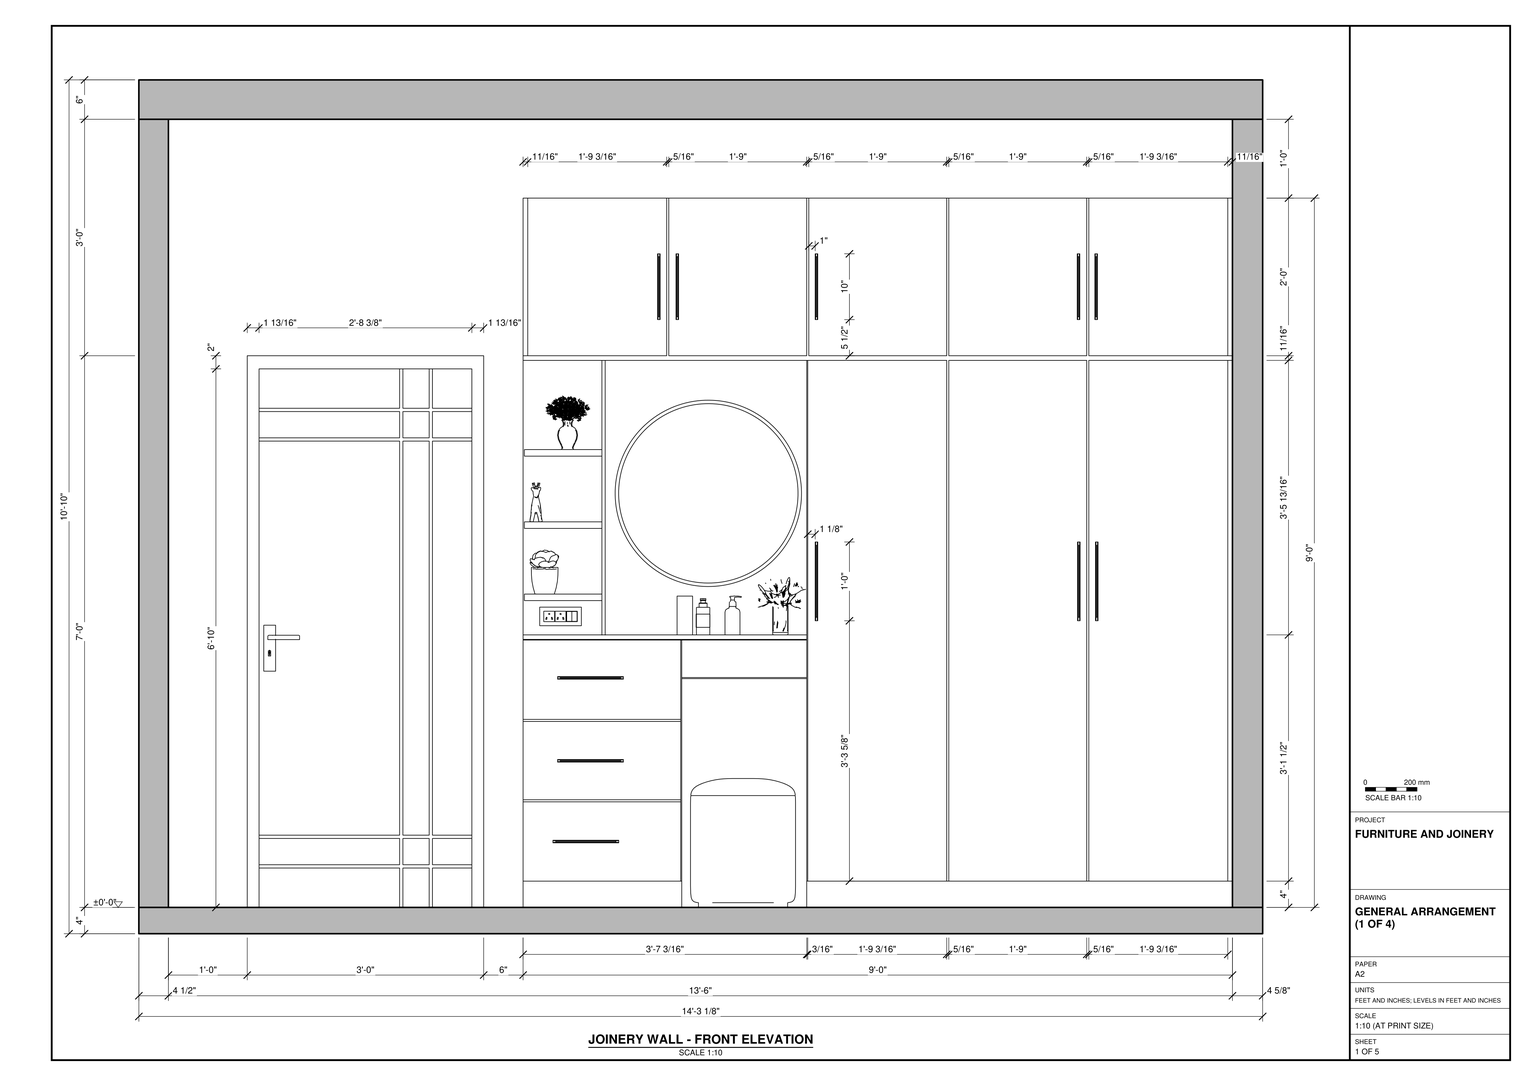
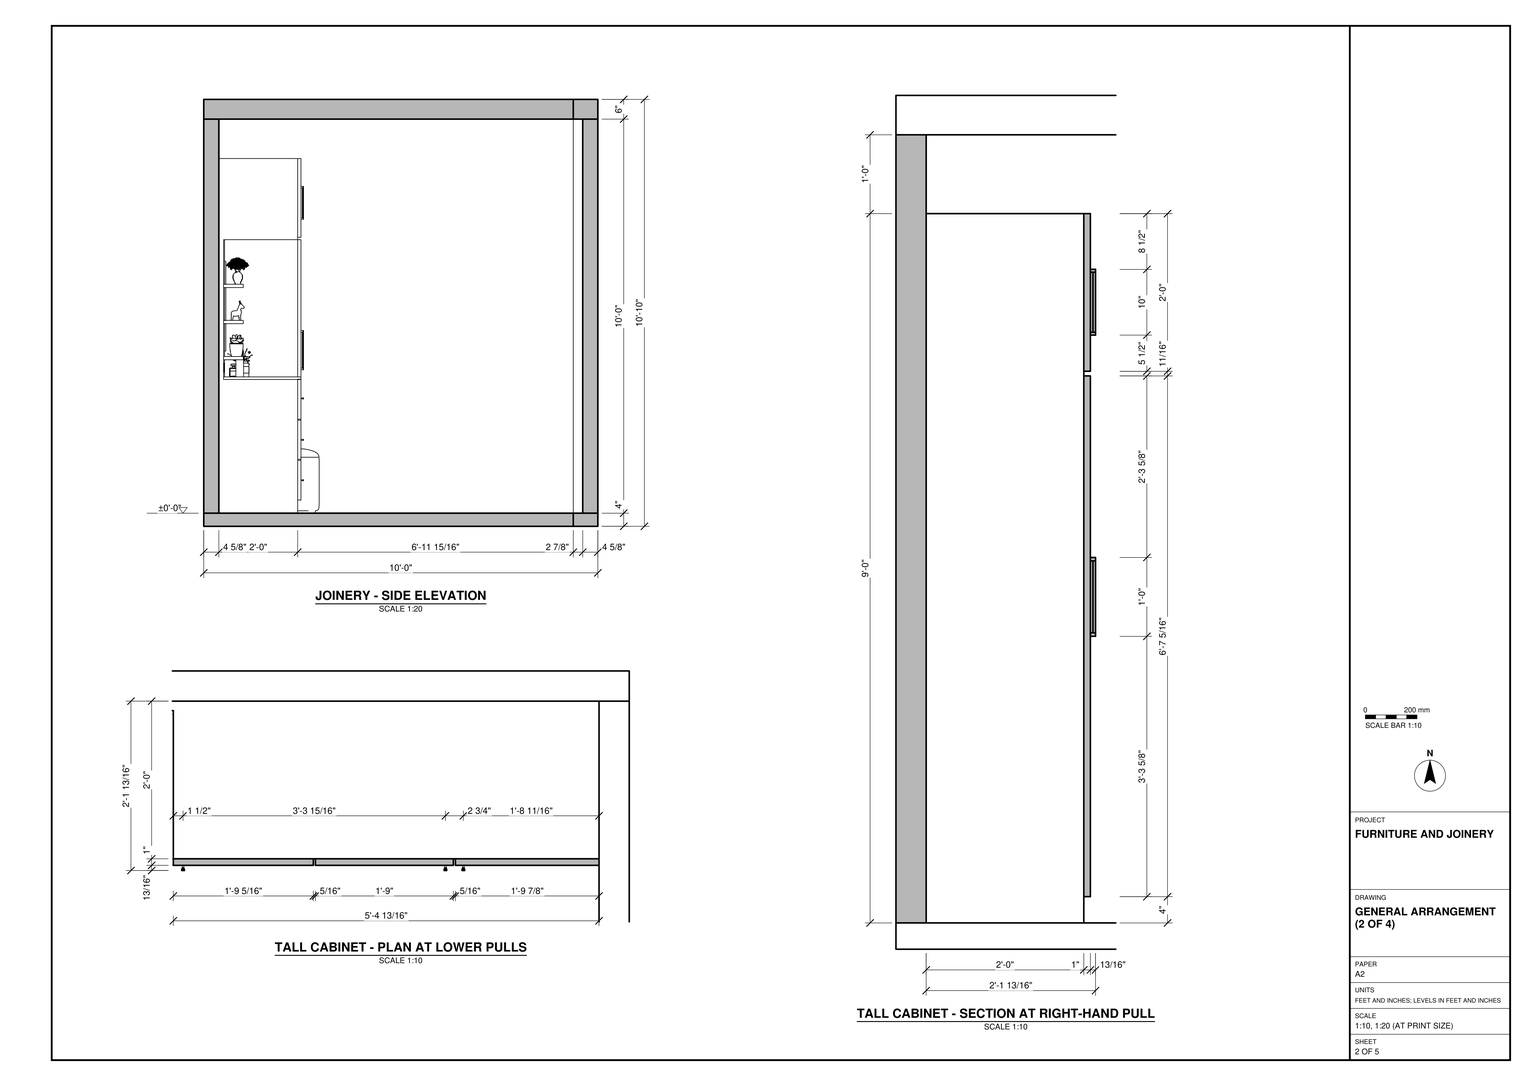
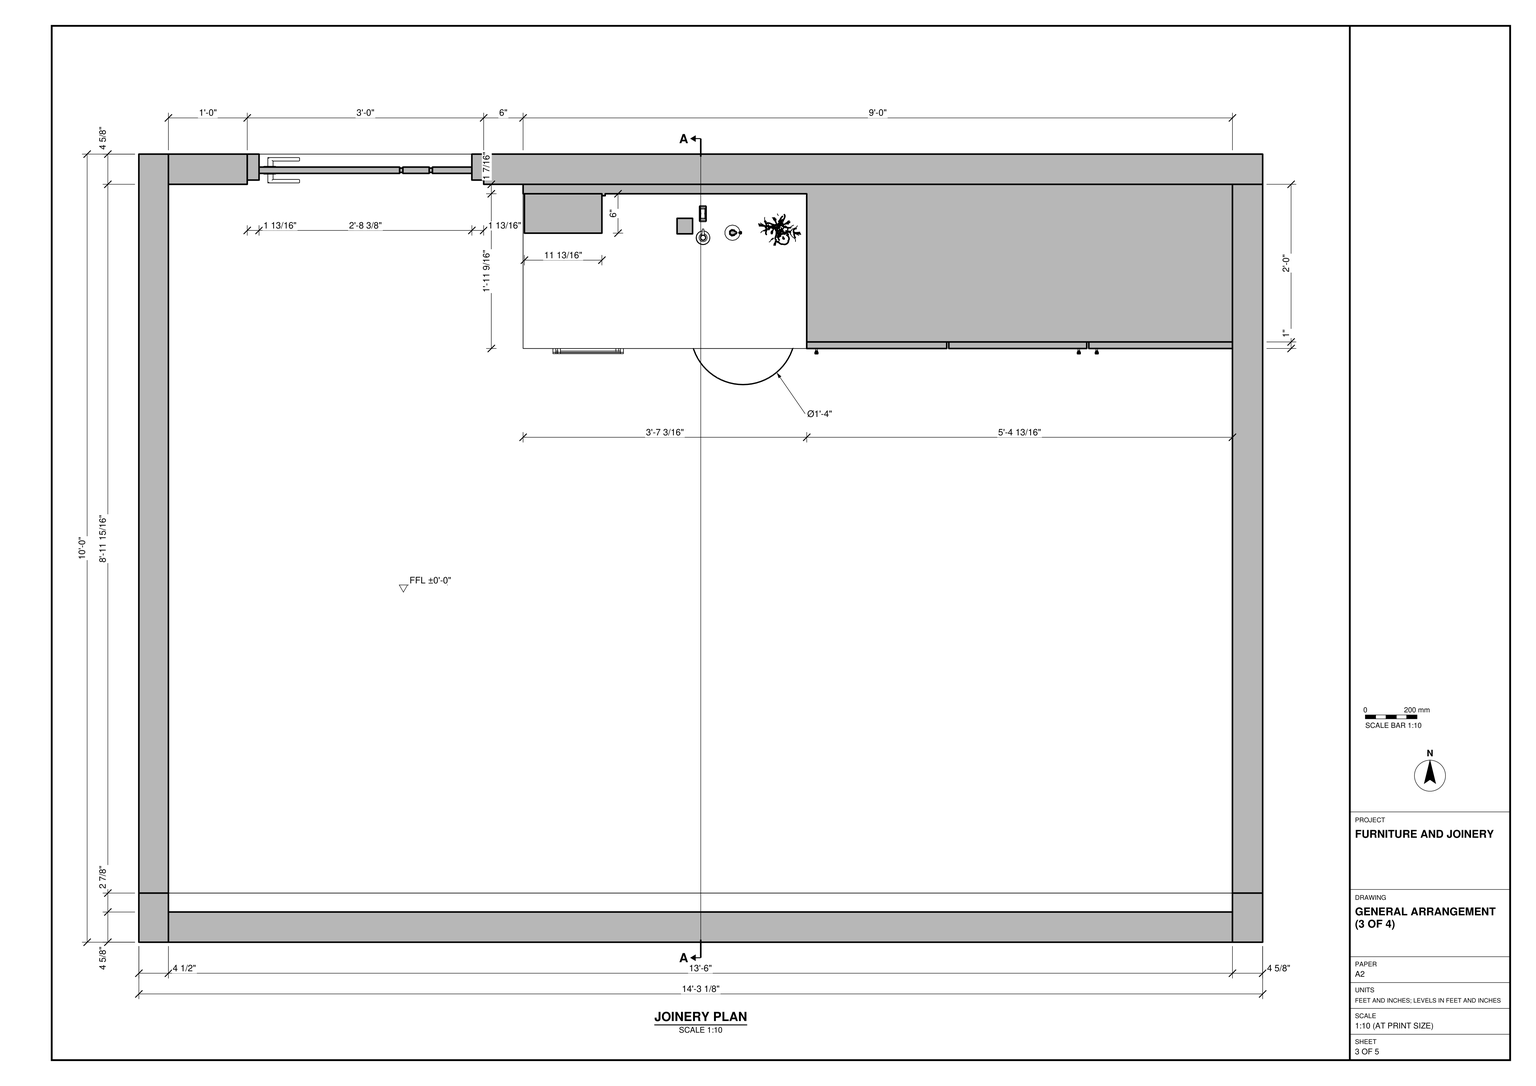
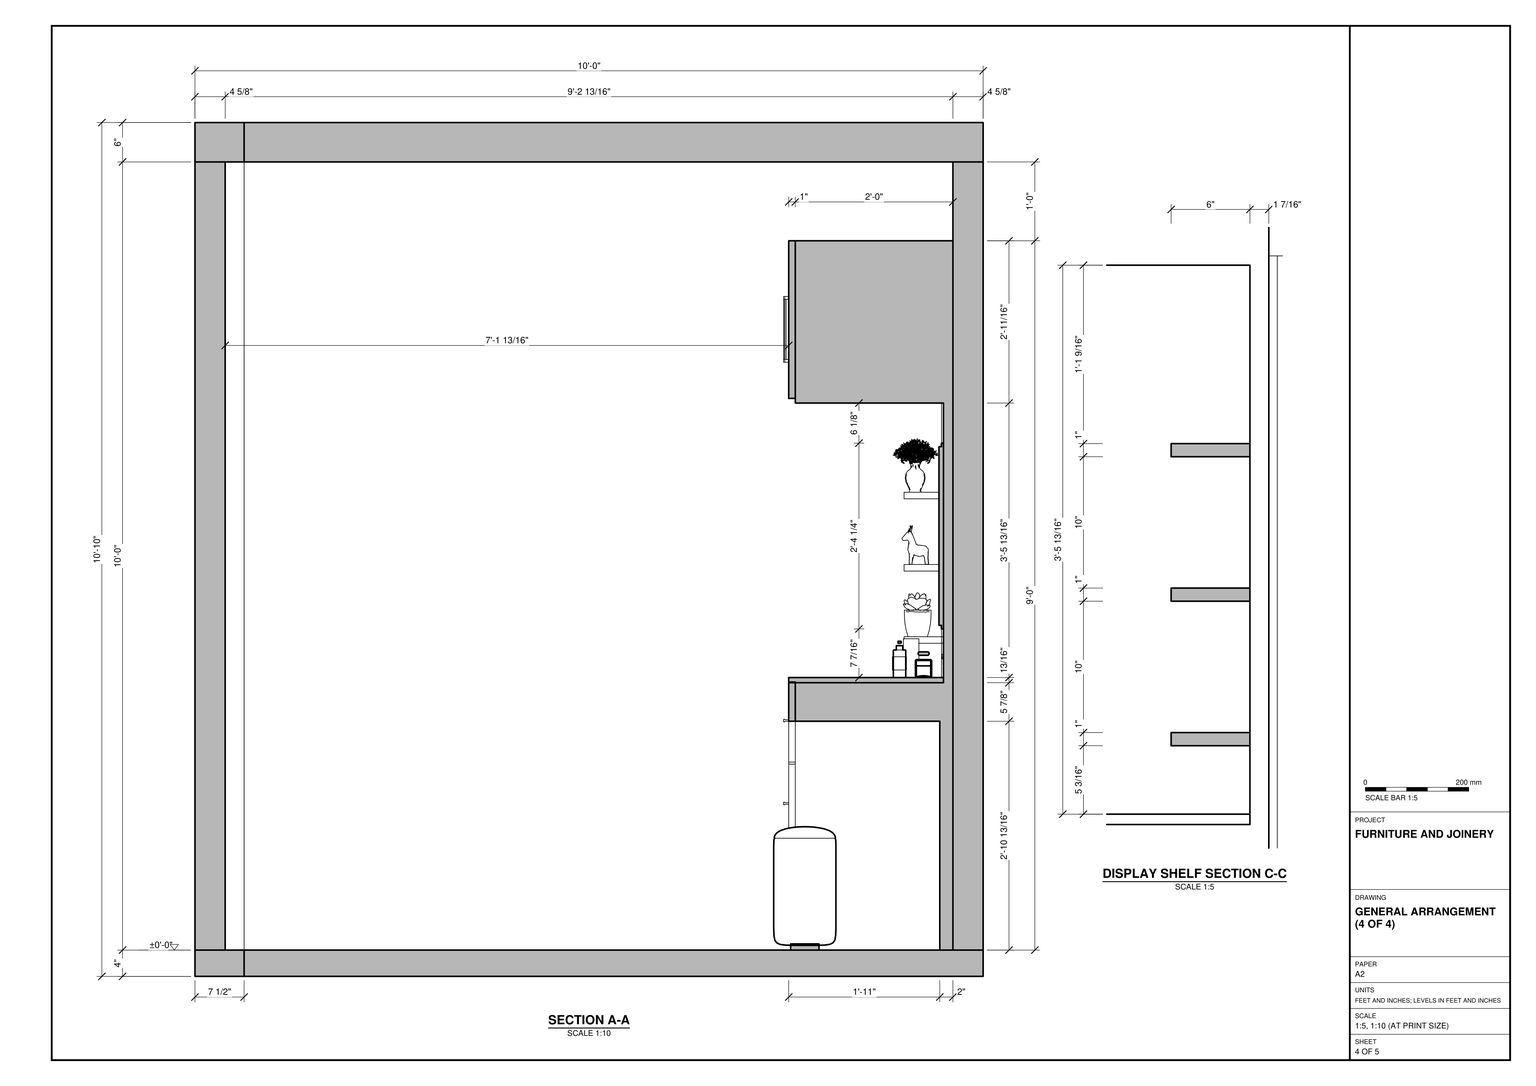
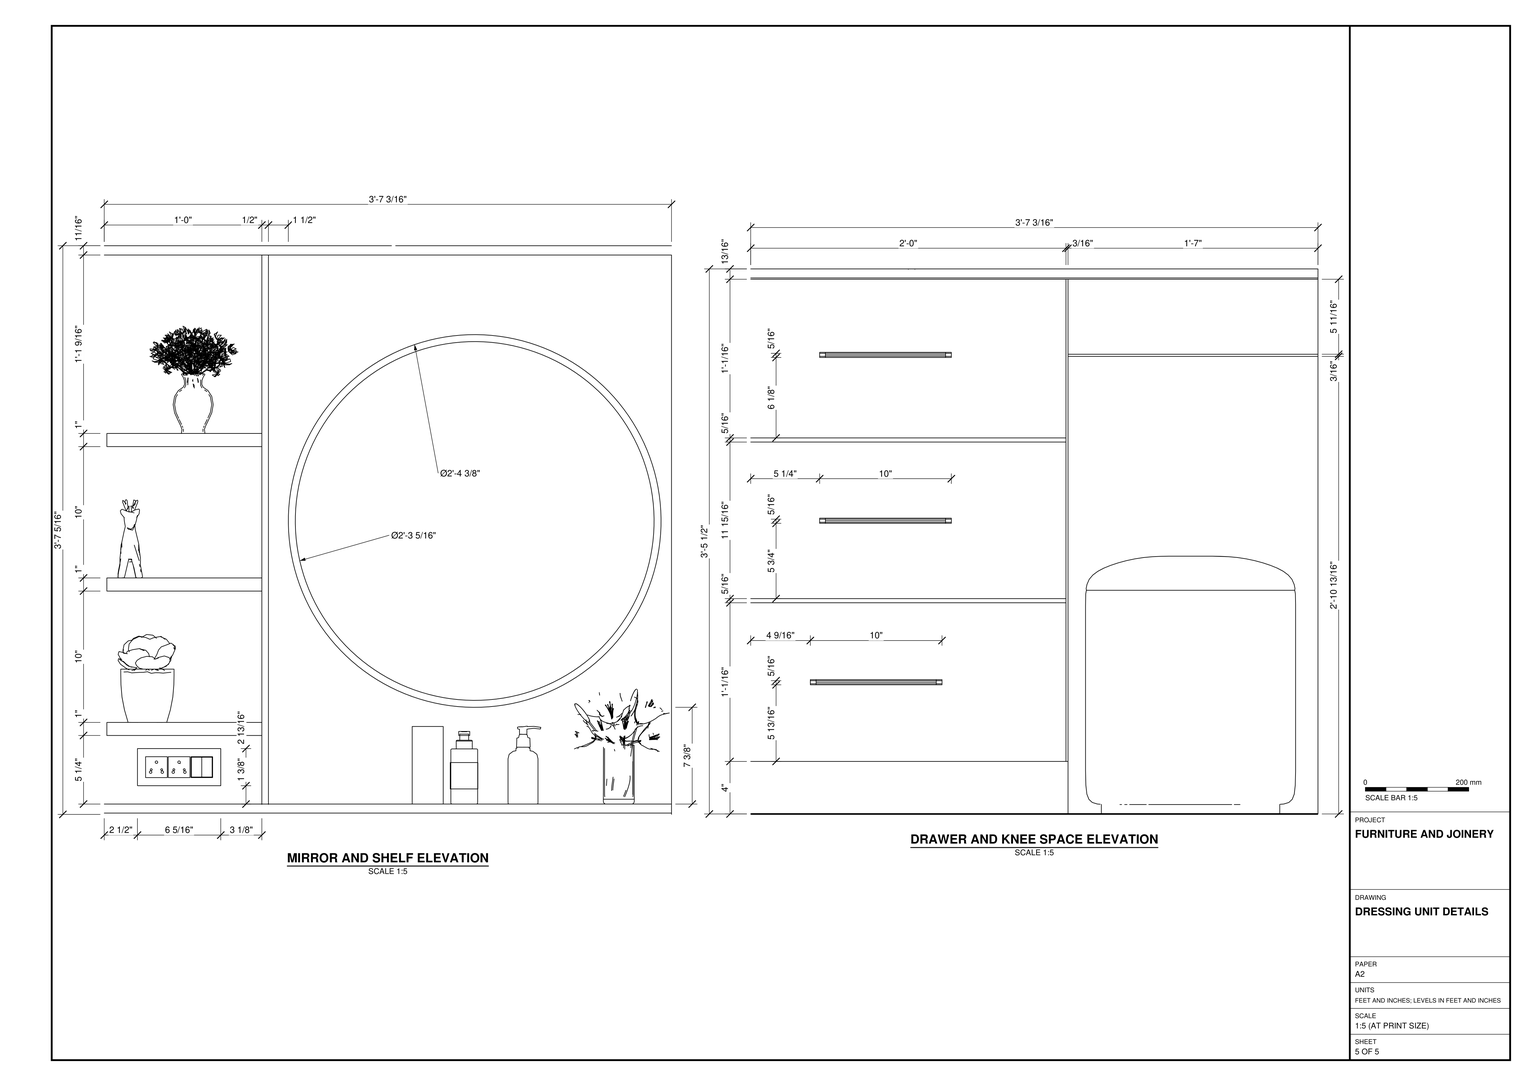
Build the joinery wall and its room shell in SketchUp using task_files/diagram_01.pdf. Work in feet and inches. The shell measures 14'-3 1/8" across the joinery wall, 10'-0" from front to back and 10'-10" overall in height. Set the finished floor at ±0'-0". Follow the plan for the wall thicknesses and the section for the floor and ceiling slabs. At the left end of the joinery wall, model the framed door with its panel divisions and lever handle.

Fit the 9'-0" cabinet run against the right wall. Carry the upper cupboards across both the dressing bay and the tall wardrobe. Below them, place the tall doors on the right and the dressing counter on the left. Include the drawer stack, knee space and round stool. Above the counter, position the circular mirror beside the narrow column of open shelves. Use the elevations and cabinet section to set the plinth, door gaps and pulls. The decor and loose items on the shelves and counter may be any suitable library components.

Keep the walls, floor slab, ceiling slab and individual joinery and furniture pieces in separate groups or components. Use components for repeated parts such as matching pulls. Save one SketchUp model as output_files/fitted_wardrobe_and_dressing_unit_with_its_room_shell.skp.

# SketchUp Ruby script. Lengths in inches.
U = 1.inch
M = Sketchup.active_model
def pt(a) = Geom::Point3d.new(a.map { |v| v * U })
def face(e, loops, mat)
  f = e.add_face(loops[0].map { |a| pt(a) })
  loops[1..].each { |l| e.add_face(l.map { |a| pt(a) }).erase! }
  f.material = f.back_material = mat if mat
  f
end
# faces: each face lists its corners as indices into pts; further lists are holes
def faces(e, pts, list, mat = nil) = list.each { |f| face(e, (f[0].is_a?(Array) ? f : [f]).map { |l| l.map { |i| pts[i] } }, mat) }
# xy, xz, yz: faces in a plane at the given z, y or x. An outline is a flat list of corners, or four numbers for a rectangle; further outlines are holes
def ring(l) = l.size == 4 ? [[l[0], l[1]], [l[2], l[1]], [l[2], l[3]], [l[0], l[3]]] : l.each_slice(2).to_a
def flat(e, list, mat, &to3) = list.each { |f| face(e, (f[0].is_a?(Array) ? f : [f]).map { |l| ring(l).map { |u, v| to3.(u, v) } }, mat) }
def xy(e, z, list, mat = nil) = flat(e, list, mat) { |x, y| [x, y, z] }
def xz(e, y, list, mat = nil) = flat(e, list, mat) { |x, z| [x, y, z] }
def yz(e, x, list, mat = nil) = flat(e, list, mat) { |y, z| [x, y, z] }
def lines(e, pts, list) = list.each { |a, b| e.add_line(pt(pts[a]), pt(pts[b])) }
# prism: a flat outline (further loops are holes) pulled along v
def prism(e, loops, v, mat = nil)
  f = face(e, loops, mat); d = Geom::Vector3d.new(v.map { |x| x * U })
  f.pushpull(f.normal.samedirection?(d) ? d.length : -d.length)
end
def box(e, o, s, mat = nil) = prism(e, [[o, [o[0] + s[0], o[1], o[2]], [o[0] + s[0], o[1] + s[1], o[2]], [o[0], o[1] + s[1], o[2]]]], [0, 0, s[2]], mat)
def at(x, y, z, deg = 0) = Geom::Transformation.translation(pt([x, y, z])) * Geom::Transformation.rotation(ORIGIN, Z_AXIS, deg.degrees)
def axes(o, x, y, z) = Geom::Transformation.new([*x, 0, *y, 0, *z, 0, *pt(o).to_a, 1])
def part(name) = M.definitions.add(name)
# library, detail: a bought-in or finely detailed component or shape, given as its bounding box
def library(name, o, s) = part(name).tap { |d| box(d.entities, o, s) }
def detail(e, o, s) = box(e.add_group.entities, o, s)
def put(e, d, t, mat = nil) = e.add_instance(d, t).tap { |i| i.material = mat if mat }
def group(e, t, mat = nil) = e.add_group.tap { |g| g.transformation = t; g.material = mat if mat }.entities
root = M.entities
M.materials.add("Manhattan Creative Coating ML 1016B 24.75cm").color = [255, 255, 255]
M.materials.add("Tiles Marble White 03 180cm").color = [241, 241, 241]
c1 = part("OuterShell")
prism(c1.entities,[[[0,0,0.08],[0,0,0.31],[0,0.59,0.31],[0,0.59,0.39],[0,0.79,0.39],[0,0.79,0],[0,0.59,0],[0,0.59,0.08]]],[0.39,0,0])
c2 = part("Cabinet pull handle")
put(c2.entities,c1,at(0,0,0))
put(c2.entities,c1,at(8.62,0,0))
g1 = group(c2.entities,at(0,0,0))
g2 = group(g1,at(0,0,0.2))
xy(g2,0,[[0.39,0.39,8.62,0.79]])
xy(g2,0.12,[[0.39,0.39,8.62,0.59]])
xy(g2,0.2,[[0.39,0.59,8.62,0.63],[0.39,0.63,8.62,0.79]])
xz(g2,0.39,[[0.39,0,8.62,0.12]])
xz(g2,0.59,[[0.39,0.12,8.62,0.2]])
xz(g2,0.79,[[0.39,0,8.62,0.2]])
yz(g2,0.39,[[0.39,0,0.39,0.12,0.59,0.12,0.59,0.2,0.79,0.2,0.79,0]])
yz(g2,8.62,[[0.39,0,0.79,0,0.79,0.2,0.59,0.2,0.59,0.12,0.39,0.12]])
g3 = group(g1,at(0,0,0.2))
xy(g3,-0.2,[[0.39,0.59,8.62,0.63],[0.39,0.63,8.62,0.79]])
xy(g3,-0.12,[[0.39,0.39,8.62,0.59]])
xy(g3,0,[[0.39,0.39,8.62,0.79]])
xz(g3,0.39,[[0.39,-0.12,8.62,0]])
xz(g3,0.59,[[0.39,-0.2,8.62,-0.12]])
xz(g3,0.79,[[0.39,-0.2,8.62,0]])
yz(g3,0.39,[[0.59,-0.2,0.79,-0.2,0.79,0,0.39,0,0.39,-0.12,0.59,-0.12]])
yz(g3,8.62,[[0.59,-0.2,0.59,-0.12,0.39,-0.12,0.39,0,0.79,0,0.79,-0.2]])
c3 = library("Potted Plant 50-24",[-2.18,-2.1,0],[4.36,4.2,6.7])
c4 = library("Vase Flowers 26-02",[-5.76,-5.9,0],[11.73,12.02,14.27])
c5 = library("Decorative Deer 209 004",[-1.58,-4.16,0],[3.36,7.25,10.63])
c6 = library("Bath Accessories 002",[-1.14,-1.17,0],[2.5,2.34,5.93])
c7 = library("Lily Flower",[-11.23,-7.61,-0.93],[19.43,20.89,23.03])
c8 = library("Component",[28.69,-29.77,58.91],[5.39,6.58,5.91])
c9 = library("Untitled",[0,0,0],[36,4.39,84])
c10 = part("Group747\#1")
p = [[0,0,0],[0,0,-1.9],[-0.92,0,-1.9],[6,-0.15,0],[-6,-0.15,0],[6,0.15,0],
  [6,0,0],[-6,0.15,0],[0.92,0,-1.9],[-6,0,0],[0,0,-3.08]]
lines(c10.entities,p,[[0,1],[1,2],[3,4],[5,6],[7,5],[1,8],[9,0],[0,6],[8,10],[4,9],[6,3],[2,10],
  [9,7]])
c11 = part("Rectangle Light")
put(c11.entities,c10,at(0,0,0))
c12 = part("Group749\#1")
p = [[0,0,0],[0,0,-1.87],[-0.91,0,-1.87],[5.9,-0.15,0],[-5.9,-0.15,0],[5.9,0.15,0],
  [5.9,0,0],[-5.9,0.15,0],[0.91,0,-1.87],[-5.9,0,0],[0,0,-3.03]]
lines(c12.entities,p,[[0,1],[1,2],[3,4],[5,6],[7,5],[1,8],[9,0],[0,6],[8,10],[4,9],[6,3],[2,10],
  [9,7]])
c13 = part("Rectangle Light\#1")
put(c13.entities,c12,at(0,0,0))
c14 = part("Group751\#1")
p = [[0,0,0],[0,0,-1.87],[-0.91,0,-1.87],[5.9,-0.15,0],[-5.9,-0.15,0],[5.9,0.15,0],
  [5.9,0,0],[-5.9,0.15,0],[0.91,0,-1.87],[-5.9,0,0],[0,0,-3.03]]
lines(c14.entities,p,[[0,1],[1,2],[3,4],[5,6],[7,5],[1,8],[9,0],[0,6],[8,10],[4,9],[6,3],[2,10],
  [9,7]])
c15 = part("Rectangle Light\#2")
put(c15.entities,c14,at(0,0,0))
c16 = part("Group753\#1")
p = [[0,0,0],[0,0,-1.87],[-0.91,0,-1.87],[5.9,-0.15,0],[-5.9,-0.15,0],[5.9,0.15,0],
  [5.9,0,0],[-5.9,0.15,0],[0.91,0,-1.87],[-5.9,0,0],[0,0,-3.03]]
lines(c16.entities,p,[[0,1],[1,2],[3,4],[5,6],[7,5],[1,8],[9,0],[0,6],[8,10],[4,9],[6,3],[2,10],
  [9,7]])
c17 = part("Rectangle Light\#3")
put(c17.entities,c16,at(0,0,0))
c18 = part("Group755\#1")
p = [[0,0,0],[0,0,-4.79],[-2.36,0,-4.79],[15.34,-0.15,0],[-15.34,-0.15,0],[15.34,0.15,0],
  [15.34,0,0],[-15.34,0.15,0],[2.36,0,-4.79],[-15.34,0,0],[0,0,-7.75]]
lines(c18.entities,p,[[0,1],[1,2],[3,4],[5,6],[7,5],[1,8],[9,0],[0,6],[8,10],[4,9],[6,3],[2,10],
  [9,7]])
c19 = part("Rectangle Light\#4")
put(c19.entities,c18,at(0,0,0))
c20 = library("Group\#8",[0,0.3125,0],[28.37,0.6875,28.375])
c21 = library("Group\#19",[0,0,0],[23.18,23.18,16.35])
c22 = library("Group\#25",[0,0,0],[16.6875,7.4375,1.35])
c23 = part("Group773\#1")
xz(c23.entities,18.59,[[-1.69,0,169.41,4]])
c24 = part("Group777\#1")
xz(c24.entities,18.59,[[164.81,4,169.41,124]])
c25 = part("Group2105\#1")
xz(c25.entities,18.59,[[-1.69,4,2.81,124]])
c26 = part("Group2135\#1")
xz(c26.entities,18.59,[[-1.69,124,169.41,130]])
c27 = part("Group770\#1")
put(c27.entities,c23,at(0,0,0))
put(c27.entities,c24,at(0,0,0))
put(c27.entities,c25,at(0,0,0))
put(c27.entities,c26,at(0,0,0))
p = [[82.5,90.4,44.71],[58.5,90.4,44.71],[101.68,90.4,44.71]]
lines(root,p,[[0,1],[2,0]])
put(root,c2,axes([79.37,90.4,103.52],[0,0,-1.11181],[0,-1,0],[-1,0,0]))
put(root,c2,axes([82.18,90.4,103.52],[0,0,-1.11181],[0,-1,0],[-1,0,0]))
put(root,c2,axes([145.95,90.4,103.52],[0,0,-1.11181],[0,-1,0],[-1,0,0]))
put(root,c2,axes([143.26,90.4,103.52],[0,0,-1.11181],[0,-1,0],[-1,0,0]))
put(root,c2,axes([103.36,90.4,103.52],[0,0,-1.11181],[0,-1,0],[-1,0,0]))
put(root,c2,axes([103.36,90.4,59.65],[0,0,-1.331],[0,-1,0],[-1,0,0]))
put(root,c2,axes([143.31,90.4,59.65],[0,0,-1.331],[0,-1,0],[-1,0,0]))
put(root,c2,axes([146.04,90.4,59.65],[0,0,-1.331],[0,-1,0],[-1,0,0]))
put(root,c2,axes([63.75,90.4,39.14],[1.11181,0,0],[0,-1,0],[0,0,-1]))
put(root,c2,axes([63.75,90.4,26.52],[1.11181,0,0],[0,-1,0],[0,0,-1]))
put(root,c2,axes([63.04,90.4,14.23],[1.11181,0,0],[0,-1,0],[0,0,-1]))
put(root,c3,at(61.74,109.97,51.71))
put(root,c4,axes([65.27,109.66,73.71],[0.5727,0,0],[0,0.5727,0],[0,0,0.5727]))
put(root,c5,axes([60.42,109.97,62.71],[0.561,0,0],[0,0.561,0],[0,0,0.561]))
put(root,c6,at(90.38,108.03,45.5))
put(root,c7,axes([98.46,107.72,45.86],[0.3933,0,0],[0,0.3933,0],[0,0,0.3933]))
put(root,c8,at(53.25,135.58,-13.42))
put(root,c9,at(16.5,115.61,4))
put(root,c11,axes([64.5,113.8125,87.28],[1,0,0],[0,-1,0],[0,0,0.13]))
put(root,c13,axes([64.6,113.8125,72.7],[1,0,0],[0,-1,0],[0,0,0.19]))
put(root,c15,axes([64.6,113.8125,61.7],[1,0,0],[0,-1,0],[0,0,0.15]))
put(root,c17,axes([64.6,113.8125,50.7],[1,0,0],[0,-1,0],[0,0,0.17]))
put(root,c19,axes([86.34,113.8125,87.28],[-1,0,0],[0,-1,0],[0,0,0.1071]))
g4 = group(root,at(27.1,0,0))
xy(g4,0,[[-27.1,0,144,120]])
xy(g4,4,[[-27.1,0,144,120]],"Tiles Marble White 03 180cm")
xz(g4,0,[[-27.1,0,144,4]])
xz(g4,120,[[-27.1,0,144,4]])
yz(g4,-27.1,[[0,0,120,4]])
yz(g4,144,[[0,0,120,4]])
g5 = group(root,at(27.1,115.4,4))
prism(g5,[[[-22.6,0,0],[-10.6,0,0],[-10.6,0,84],[25.4,0,84],[25.4,0,0],[144,0,0],[144,0,120],[-22.6,0,120]]],[0,4.6,0])
g6 = group(root,at(166.5,0,4))
box(g6,[0,0,0],[4.6,115.4,120])
g7 = group(root,at(58.5,91.4,4),"Manhattan Creative Coating ML 1016B 24.75cm")
xy(g7,0,[[0,0,0,24,108,24,108,0,43.18,0,43.18,22,24.16,22,24.16,0]])
xy(g7,34.84,[[24.16,0,43.18,22]])
xy(g7,40.71,[[0,0,43.18,0,43.18,22.5625,12.5,22.5625,12.5,22.26,12,22.26,12,22.5625,0,22.5625]])
xy(g7,46.71,[[0.2,16.5625,12,22.5625]])
xy(g7,47.71,[[0.2,16.5625,12,22.5625]])
xy(g7,57.71,[[0.2,16.5625,12,22.5625]])
xy(g7,58.71,[[0.2,16.5625,12,22.5625]])
xy(g7,68.71,[[0.2,16.5625,12,22.5625]])
xy(g7,69.71,[[0.2,16.5625,12,22.5625]])
xy(g7,83.29,[[0,0,0,22.5625,12,22.5625,12,22.26,12.5,22.26,12.5,22.5625,43.18,22.5625,43.18,0]])
xy(g7,108,[[0,0,108,24]])
xz(g7,0,[[0,0,24.16,4],[43.18,0,108,4],[0,4,24.16,4,24.16,34.84,43.18,34.84,43.18,4,108,4,108,108,0,108,0,83.29,43.18,83.29,43.18,40.71,0,40.71]])
xz(g7,16.5625,[[0.2,46.71,12,47.71],[0.2,57.71,12,58.71],[0.2,68.71,12,69.71]])
xz(g7,22,[[24.16,0,43.18,34.84]])
xz(g7,22.26,[[12,40.71,12.5,83.29]])
xz(g7,22.5625,[[0,40.71,12,40.71,12,46.71,0.2,46.71,0.2,47.71,12,47.71,12,57.71,0.2,57.71,0.2,58.71,12,58.71,12,68.71,0.2,68.71,0.2,69.71,12,69.71,12,83.29,0,83.29],[12.5,40.71,43.18,83.29],[0.2,46.71,12,47.71],[0.2,57.71,12,58.71],[0.2,68.71,12,69.71]])
xz(g7,24,[[0,0,108,108]])
yz(g7,0,[[0,0,0,40.71,22.5625,40.71,22.5625,83.29,0,83.29,0,108,24,108,24,0]],"Manhattan Creative Coating ML 1016B 24.75cm")
yz(g7,0.2,[[16.5625,46.71,22.5625,47.71],[16.5625,57.71,22.5625,58.71],[16.5625,68.71,22.5625,69.71]])
yz(g7,12,[[22.26,40.71,22.5625,46.71],[16.5625,46.71,22.26,47.71],[22.26,46.71,22.5625,47.71],[22.26,47.71,22.5625,57.71],[16.5625,57.71,22.26,58.71],
  [22.26,57.71,22.5625,58.71],[22.26,58.71,22.5625,68.71],[16.5625,68.71,22.26,69.71],[22.26,68.71,22.5625,69.71],[22.26,69.71,22.5625,83.29]])
yz(g7,12.5,[[22.26,40.71,22.5625,83.29]])
yz(g7,24.16,[[0,0,22,34.84]])
yz(g7,43.18,[[0,0,22,34.84],[0,40.71,22.5625,83.29]])
yz(g7,108,[[0,0,24,108]])
g8 = group(root,at(58.5,90.4,8),"Manhattan Creative Coating ML 1016B 24.75cm")
box(g8,[64.82,0,80],[21,1,24])
box(g8,[43.5,0,80],[21,1,24])
box(g8,[22.18,0,80],[21,1,24])
box(g8,[64.82,0,0],[21,1,79.29])
xy(g8,0,[[0,0,24.16,1],[43.18,0,64.5,1],[86.13,0,108,1]])
xy(g8,12.08,[[0,0,24,1]])
xy(g8,12.39,[[0,0,24,1]])
xy(g8,24.31,[[0,0,24,1]])
xy(g8,24.63,[[0,0,24,1]])
xy(g8,30.84,[[24.16,0,43.18,1]])
xy(g8,36.71,[[0,0,43.18,1]])
xy(g8,79.29,[[43.18,0,43.34,1],[43.34,0,43.5,1],[43.5,0,64.5,1],[86.13,0,107.29,1],[107.29,0,108,1]])
xy(g8,80,[[0,0,0.71,1],[0.71,0,21.87,1],[86.13,0,107.29,1],[107.29,0,108,1]])
xy(g8,104,[[0,0,21.87,1],[86.13,0,108,1]])
xz(g8,0,[[0,0,24,12.08],[24,0,24.16,36.71],[43.18,0,43.34,79.29],[43.34,0,64.5,79.29],[86.13,0,107.29,79.29],
  [107.29,0,108,79.29],[0,12.39,24,24.31],[0,24.63,24,36.71],[24.16,30.84,43.18,31],[24.16,31,43.18,36.71],
  [0,80,0.71,104],[0.71,80,21.87,104],[86.13,80,107.29,104],[107.29,80,108,104]])
xz(g8,1,[[0,0,0,12.08,24,12.08,24,12.39,0,12.39,0,24.31,24,24.31,24,24.63,0,24.63,0,36.71,43.18,36.71,43.18,79.29,64.5,79.29,64.5,0,43.18,0,43.18,30.84,24.16,30.84,24.16,0],[86.13,0,108,79.29],[0,80,21.87,104],[86.13,80,108,104]])
yz(g8,0,[[0,0,1,12.08],[0,12.39,1,24.31],[0,24.63,1,36.71],[0,80,1,104]])
yz(g8,21.87,[[0,80,1,104]])
yz(g8,24,[[0,12.08,1,12.39],[0,24.31,1,24.63]])
yz(g8,24.16,[[0,0,1,30.84]])
yz(g8,43.18,[[0,0,1,30.84],[0,36.71,1,79.29]])
yz(g8,64.5,[[0,0,1,79.29]])
yz(g8,86.13,[[0,0,1,79.29],[0,80,1,104]])
yz(g8,108,[[0,0,1,79.29],[0,80,1,104]])
p = [[0,1,79.29],[0,1,80],[0.71,1,79.29],[21.87,1,79.29],[108,1,80],[108,1,79.29],
  [86.13,1,0],[85.82,1,0],[22.03,1,79.29],[22.18,1,79.29],[43.18,1,79.29]]
lines(g8,p,[[0,1],[0,2],[2,3],[4,5],[6,7],[3,8],[8,9],[9,10]])
g9 = group(root,at(58.5,91.4,44.71),"Manhattan Creative Coating ML 1016B 24.75cm")
prism(g9,[[[43.18,0,0],[43.18,22.5625,0],[43.18,22.5625,0.79],[43.18,-1,0.79],[43.18,-1,0.1],[43.18,0,0.1]]],[-43.18,0,0])
put(root,c20,at(72.52,112.96,52.86))
put(root,c21,axes([83.99,84.86,4],[0.69,0,0],[0,0.69,0],[0,0,1.2006]))
g10 = group(root,at(0,0,4))
box(g10,[0,0,0],[4.5,120,120])
g11 = group(root,at(4.5,0,4))
box(g11,[0,0,0],[162,4.6,120])
g12 = group(root,at(0,0,124))
box(g12,[0,0,0],[171.1,120,6])
put(root,c22,axes([61.03,114.23,46.89],[0.38,0,0],[0,0,0.38],[0,-0.38,0]))
put(root,c27,at(1.69,-11.11,0))
